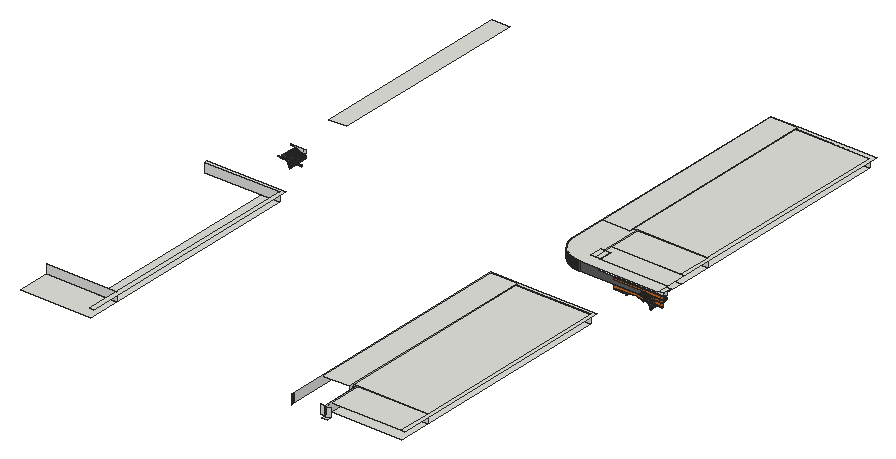
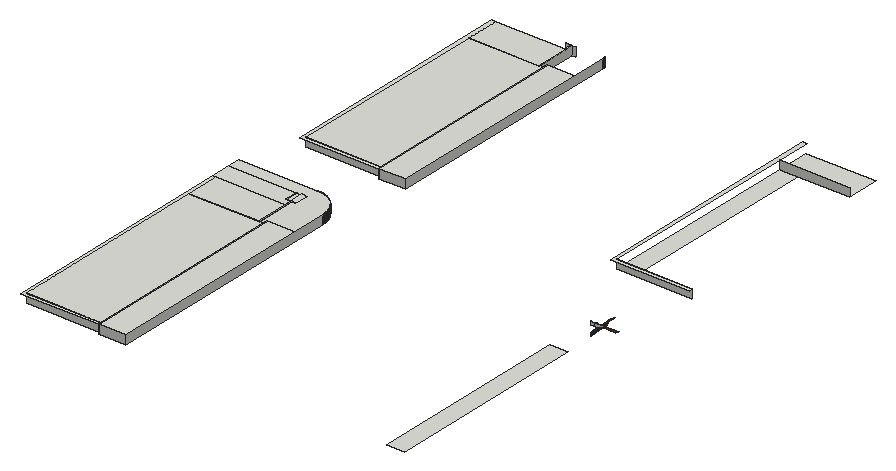
# SketchUp Ruby script. Lengths in inches.
U = 1.inch
M = Sketchup.active_model
def pt(a) = Geom::Point3d.new(a.map { |v| v * U })
def face(e, loops, mat)
  f = e.add_face(loops[0].map { |a| pt(a) })
  loops[1..].each { |l| e.add_face(l.map { |a| pt(a) }).erase! }
  f.material = f.back_material = mat if mat
  f
end
# faces: each face lists its corners as indices into pts; further lists are holes
def faces(e, pts, list, mat = nil) = list.each { |f| face(e, (f[0].is_a?(Array) ? f : [f]).map { |l| l.map { |i| pts[i] } }, mat) }
# xy, xz, yz: faces in a plane at the given z, y or x. An outline is a flat list of corners, or four numbers for a rectangle; further outlines are holes
def ring(l) = l.size == 4 ? [[l[0], l[1]], [l[2], l[1]], [l[2], l[3]], [l[0], l[3]]] : l.each_slice(2).to_a
def flat(e, list, mat, &to3) = list.each { |f| face(e, (f[0].is_a?(Array) ? f : [f]).map { |l| ring(l).map { |u, v| to3.(u, v) } }, mat) }
def xy(e, z, list, mat = nil) = flat(e, list, mat) { |x, y| [x, y, z] }
def xz(e, y, list, mat = nil) = flat(e, list, mat) { |x, z| [x, y, z] }
def yz(e, x, list, mat = nil) = flat(e, list, mat) { |y, z| [x, y, z] }
def lines(e, pts, list) = list.each { |a, b| e.add_line(pt(pts[a]), pt(pts[b])) }
# prism: a flat outline (further loops are holes) pulled along v
def prism(e, loops, v, mat = nil)
  f = face(e, loops, mat); d = Geom::Vector3d.new(v.map { |x| x * U })
  f.pushpull(f.normal.samedirection?(d) ? d.length : -d.length)
end
def box(e, o, s, mat = nil) = prism(e, [[o, [o[0] + s[0], o[1], o[2]], [o[0] + s[0], o[1] + s[1], o[2]], [o[0], o[1] + s[1], o[2]]]], [0, 0, s[2]], mat)
def at(x, y, z, deg = 0) = Geom::Transformation.translation(pt([x, y, z])) * Geom::Transformation.rotation(ORIGIN, Z_AXIS, deg.degrees)
def axes(o, x, y, z) = Geom::Transformation.new([*x, 0, *y, 0, *z, 0, *pt(o).to_a, 1])
def part(name) = M.definitions.add(name)
# library, detail: a bought-in or finely detailed component or shape, given as its bounding box
def library(name, o, s) = part(name).tap { |d| box(d.entities, o, s) }
def detail(e, o, s) = box(e.add_group.entities, o, s)
def put(e, d, t, mat = nil) = e.add_instance(d, t).tap { |i| i.material = mat if mat }
def group(e, t, mat = nil) = e.add_group.tap { |g| g.transformation = t; g.material = mat if mat }.entities
root = M.entities
M.materials.add("[0041_Chocolate]").color = [210, 105, 30]
M.materials.add("[Color M06]").color = [84, 84, 84]
xy(root,385.02,[[1533.33,971.36,1577.46,972.36],[2230.65,971.36,2260.14,972.36],[2287.96,971.36,2332.08,972.36]],"[0041_Chocolate]")
xy(root,386.9375,[[1528.37,971.36,1577.46,972.36],[2230.65,971.36,2265.11,972.36],[2282.99,971.36,2332.08,972.36]],"[0041_Chocolate]")
xy(root,391.89,[[2230.65,971.36,2332.08,972.36]],"[0041_Chocolate]")
xy(root,393.8125,[[2230.65,971.36,2332.08,972.36]],"[0041_Chocolate]")
xy(root,395.26,[[2230.65,993.35,2309.9,1001.16]])
xy(root,398.77,[[2230.65,971.36,2332.08,972.36]],"[0041_Chocolate]")
xy(root,400.6875,[[2230.65,971.36,2332.08,972.36]],"[0041_Chocolate]")
xy(root,402.64,[[2146.71,312.8125,2158.24,321.34],[1496.21,337.5625,1643.23,406.38],[2146.71,337.5625,2293.73,406.38],[2145.53,399.07,2146.71,406.38],[1606.23,406.38,1643.23,830.91],
  [2137,406.38,2145.53,830.91],[2145.53,406.38,2256.73,830.91],[2256.73,406.38,2293.73,830.91],[2230.65,991.23,2291.86,993.35],[2323.46,993.35,2326.17,993.35,2326.17,1028.46,2179.15,1028.46,2179.15,1012.23,2190.68,1012.23,2190.68,996.48,2230.65,996.48,2230.65,1003.71,2323.46,1003.71],
  [2230.65,993.35,2323.46,1003.71],[2169.44,996.48,2179.15,1003.71],[2179.15,996.48,2190.68,1003.71],[2169.44,1003.71,2179.15,1012.23],[2179.15,1003.71,2190.68,1012.23],
  [2179.15,1028.46,2326.17,1097.28],[2177.96,1089.96,2179.15,1097.28],[1534.54,1097.28,1571.54,1521.81],[2169.44,1097.28,2177.96,1521.81],[2177.96,1097.28,2289.17,1521.81],
  [2289.17,1097.28,2326.17,1521.81]])
xy(root,402.64,[[2168.39,958.64,2166.9,958.66,2165.41,958.72,2163.93,958.82,2162.44,958.96,2160.96,959.13,2159.49,959.34,2158.02,959.6,2156.5625,959.89,2155.11,960.22,2153.67,960.58,2152.23,960.99,2150.8125,961.43,2149.4,961.91,2148,962.42,2146.62,962.97,2145.25,963.5625,2143.9,964.1875,2142.5625,964.84,2141.25,965.54,2139.95,966.27,2138.67,967.03,2137.41,967.82,2136.17,968.65,2134.95,969.51,2133.76,970.4,2132.59,971.32,2131.44,972.27,2130.32,973.26,2129.23,974.27,2128.16,975.31,2127.125,976.37,2126.11,977.47,2125.13,978.59,2124.18,979.73,2123.26,980.9,2122.37,982.09,2121.51,983.31,2120.68,984.55,2119.89,985.81,2119.125,987.09,2118.4,988.39,2117.7,989.71,2117.04,991.04,2116.42,992.39,2115.83,993.76,2115.28,995.14,2114.77,996.54,2114.29,997.95,2113.85,999.375,2113.44,1000.81,2113.07,1002.25,2112.75,1003.7,2112.46,1005.16,2112.2,1006.63,2111.99,1008.11,2111.8125,1009.58,2111.68,1011.07,2111.58,1012.55,2111.52,1014.04,2111.5,1015.53,2111.5,1529.04,2169.44,1529.04,2169.44,996.48,2190.68,996.48,2190.68,978.84,2230.65,978.84,2230.65,991.23,2291.86,991.23,2291.86,958.64]],"[Color M06]")
xy(root,405.64,[[2230.65,971.36,2332.08,972.36]],"[0041_Chocolate]")
xy(root,411.82,[[2230.65,972.36,2332.08,993.35]])
xy(root,421.25,[[2145.53,321.34,2146.71,406.38],[2146.71,321.34,2148.59,321.34,2148.59,336.27,2293.73,336.27,2293.73,406.38,2146.71,406.38],[1643.23,336.27,1650.02,336.27,1650.02,838.14,1486.5,838.14,1486.5,830.91,1643.23,830.91],[2293.73,336.27,2300.52,336.27,2300.52,838.14,2137,838.14,2137,830.91,2293.73,830.91],[2079.07,397.86,2137,838.14],
  [2137,406.38,2293.73,830.91],[2168.39,958.64,2332.96,958.64,2332.96,983.34,2169.44,983.34,2169.44,1012.23,2177.96,1012.23,2177.96,1097.28,2169.44,1097.28,2169.44,1088.75,2111.5,1088.75,2111.5,1015.53,2111.52,1014.04,2111.58,1012.55,2111.68,1011.07,2111.8125,1009.58,2111.99,1008.11,2112.2,1006.63,2112.46,1005.16,2112.75,1003.7,2113.07,1002.25,2113.44,1000.81,2113.85,999.375,2114.29,997.95,2114.77,996.54,2115.28,995.14,2115.83,993.76,2116.42,992.39,2117.04,991.04,2117.7,989.71,2118.4,988.39,2119.125,987.09,2119.89,985.81,2120.68,984.55,2121.51,983.31,2122.37,982.09,2123.26,980.9,2124.18,979.73,2125.13,978.59,2126.11,977.47,2127.125,976.37,2128.16,975.31,2129.23,974.27,2130.32,973.26,2131.44,972.27,2132.59,971.32,2133.76,970.4,2134.95,969.51,2136.17,968.65,2137.41,967.82,2138.67,967.03,2139.95,966.27,2141.25,965.54,2142.5625,964.84,2143.9,964.1875,2145.25,963.5625,2146.62,962.97,2148,962.42,2149.4,961.91,2150.8125,961.43,2152.23,960.99,2153.67,960.58,2155.11,960.22,2156.5625,959.89,2158.02,959.6,2159.49,959.34,2160.96,959.13,2162.44,958.96,2163.93,958.82,2165.41,958.72,2166.9,958.66],[2169.44,983.34,2181.03,1012.23],[2181.03,983.34,2190.68,1012.23],[2190.68,983.34,2332.96,983.34,2332.96,1027.17,2181.03,1027.17,2181.03,1012.23,2190.68,1012.23],
  [2177.96,1012.23,2179.15,1097.28],[2179.15,1012.23,2181.03,1012.23,2181.03,1027.17,2326.17,1027.17,2326.17,1097.28,2179.15,1097.28],[2326.17,1027.17,2332.96,1027.17,2332.96,1529.04,2169.44,1529.04,2169.44,1521.81,2326.17,1521.81],[2111.5,1088.75,2169.44,1529.04],[2169.44,1097.28,2326.17,1521.81]])
xz(root,321.34,[[2137,402.64,2145.53,421.25],[2145.53,402.64,2146.71,421.25],[2146.71,402.64,2148.59,421.25],[2148.59,402.64,2158.24,421.25]])
xz(root,406.38,[[1496.21,402.64,1643.23,421.25],[2137,402.64,2145.53,421.25],[2145.53,402.64,2146.71,421.25],[2146.71,402.64,2293.73,421.25]])
xz(root,830.91,[[1486.5,402.64,1643.23,421.25],[2137,402.64,2293.73,421.25]])
xz(root,838.14,[[2079.07,402.64,2137,421.25]])
xz(root,971.36,[[2230.65,386.9375,2265.11,386.9375,2269.94,388.23,2278.13,388.24,2282.99,386.9375,2332.08,386.9375,2332.08,391.89,2230.65,391.89],[2230.65,393.8125,2332.08,398.77],[2230.65,400.6875,2332.08,405.64]],"[0041_Chocolate]")
xz(root,972.36,[[2230.65,405.64,2332.08,407.5625],[2230.65,407.5625,2332.08,411.82],[2230.65,411.82,2332.08,412.52]])
xz(root,972.36,[[1533.33,385.02,1577.46,385.02,1577.46,386.9375,1528.37,386.9375,1531.41,386.125],[2230.65,385.02,2260.14,385.02,2262.03,386.11,2265.11,386.9375,2230.65,386.9375],[2287.96,385.02,2332.08,385.02,2332.08,386.9375,2282.99,386.9375,2286.04,386.125],[2230.65,391.89,2332.08,393.8125],[2230.65,398.77,2332.08,400.6875]],"[0041_Chocolate]")
xz(root,993.35,[[1555.27,395.26,1562.99,395.26,1562.99,402.64,1537.23,402.64,1537.91,402.625,1538.58,402.6,1539.25,402.56,1539.92,402.49,1540.59,402.41,1541.26,402.32,1541.93,402.2,1542.59,402.07,1543.25,401.92,1543.9,401.76,1544.55,401.57,1545.19,401.375,1545.83,401.16,1546.46,400.92,1547.09,400.67,1547.71,400.41,1548.32,400.125,1548.93,399.83,1549.52,399.51,1550.11,399.18,1550.69,398.84,1551.26,398.48,1551.82,398.1,1552.37,397.72,1552.91,397.3125,1553.44,396.89,1553.96,396.46,1554.47,396.02,1554.96,395.5625],[1562.99,395.26,1568.84,402.64],[2230.65,395.26,2309.9,395.26,2309.59,395.5625,2309.09,396.02,2308.59,396.46,2308.07,396.89,2307.54,397.3125,2307,397.72,2306.45,398.1,2305.89,398.48,2305.32,398.84,2304.74,399.18,2304.15,399.51,2303.55,399.83,2302.95,400.125,2302.33,400.41,2301.71,400.67,2301.09,400.92,2300.46,401.16,2299.82,401.375,2299.17,401.57,2298.52,401.76,2297.87,401.92,2297.21,402.07,2296.55,402.2,2295.89,402.32,2295.22,402.41,2294.55,402.49,2293.88,402.56,2293.2,402.6,2292.53,402.625,2291.86,402.64,2230.65,402.64],[2309.9,395.26,2317.62,395.26,2317.62,402.64,2291.86,402.64,2292.53,402.625,2293.2,402.6,2293.88,402.56,2294.55,402.49,2295.22,402.41,2295.89,402.32,2296.55,402.2,2297.21,402.07,2297.87,401.92,2298.52,401.76,2299.17,401.57,2299.82,401.375,2300.46,401.16,2301.09,400.92,2301.71,400.67,2302.33,400.41,2302.95,400.125,2303.55,399.83,2304.15,399.51,2304.74,399.18,2305.32,398.84,2305.89,398.48,2306.45,398.1,2307,397.72,2307.54,397.3125,2308.07,396.89,2308.59,396.46,2309.09,396.02,2309.59,395.5625],[2317.62,395.26,2323.46,402.64],
  [2230.65,402.64,2317.62,411.82]])
xz(root,1012.23,[[2169.44,402.64,2177.96,421.25],[2177.96,402.64,2179.15,421.25],[2179.15,402.64,2181.03,421.25],[2181.03,402.64,2190.68,421.25]])
xz(root,1097.28,[[2169.44,402.64,2177.96,421.25],[2177.96,402.64,2179.15,421.25],[2179.15,402.64,2326.17,421.25]])
xz(root,1521.81,[[2169.44,402.64,2326.17,421.25]])
xz(root,1529.04,[[2111.5,402.64,2169.44,421.25]])
yz(root,2079.07,[[324.64,402.64,838.14,421.25]])
yz(root,2111.5,[[1015.53,402.64,1529.04,421.25]])
yz(root,2137,[[397.86,402.64,406.38,421.25],[406.38,402.64,830.91,421.25],[830.91,402.64,838.14,421.25]])
yz(root,2146.71,[[321.34,402.64,406.38,421.25]])
yz(root,2169.44,[[1088.75,402.64,1097.28,421.25],[1097.28,402.64,1521.81,421.25],[1521.81,402.64,1529.04,421.25]])
yz(root,2179.15,[[1012.23,402.64,1097.28,421.25]])
yz(root,2190.68,[[983.34,402.64,1012.23,421.25]])
yz(root,2230.65,[[991.23,395.26,993.35,402.64],[993.35,395.26,996.48,402.64]])
p = [[1562.56,958.64,381.57],[1562.56,993.35,381.57],[1562.67,993.35,380.9],[1562.67,958.64,380.9],[2317.19,958.64,381.57],[2317.19,993.35,381.57],
  [2317.3,993.35,380.9],[2317.3,958.64,380.9],[1562.67,1001.16,380.9],[1562.56,1001.16,381.57],[2317.3,1001.16,380.9],[2317.19,1001.16,381.57],
  [1562.43,958.64,382.23],[1562.43,993.35,382.23],[2317.05,958.64,382.23],[2317.05,993.35,382.23],[1562.43,1001.16,382.23],[2317.05,1001.16,382.23],
  [2260.14,986.55,385.02],[2260.14,972.36,385.02],[2260.14,971.36,385.02],[2254.94,971.36,382.01],[2254.94,986.55,382.01],[2293.13,986.55,382.03],
  [2293.13,971.36,382.03],[2287.96,971.36,385.02],[2287.96,972.36,385.02],[2287.96,986.55,385.02],[1562.28,958.64,382.89],[1562.28,993.35,382.89],
  [2316.9,958.64,382.89],[2316.9,993.35,382.89],[1562.28,1001.16,382.89],[2316.9,1001.16,382.89],[1562.11,958.64,383.54],[1562.11,993.35,383.54],
  [2316.74,958.64,383.54],[2316.74,993.35,383.54],[1562.11,1001.16,383.54],[2316.74,1001.16,383.54],[1561.93,958.64,384.19],[1561.93,993.35,384.19],
  [1562.09,993.35,383.64],[2316.56,958.64,384.19],[2316.56,993.35,384.19],[2316.71,993.35,383.64],[1562.09,1001.16,383.64],[2316.71,1001.16,383.64],
  [1561.93,1001.16,384.19],[2316.56,1001.16,384.19],[1561.73,958.64,384.84],[1561.73,993.35,384.84],[2316.36,958.64,384.84],[2316.36,993.35,384.84],
  [1561.73,1001.16,384.84],[2316.36,1001.16,384.84],[1561.51,958.64,385.47],[1561.51,993.35,385.47],[2316.14,958.64,385.47],[2316.14,993.35,385.47],
  [1561.51,1001.16,385.47],[2316.14,1001.16,385.47],[2262.03,972.36,386.11],[2262.03,986.55,386.11],[2286.04,972.36,386.125],[2286.04,986.55,386.125],
  [1561.28,958.64,386.11],[1561.28,993.35,386.11],[1561.41,993.35,385.76],[2315.91,958.64,386.11],[2315.91,993.35,386.11],[2316.03,993.35,385.76],
  [1561.41,1001.16,385.76],[2316.03,1001.16,385.76],[1561.28,1001.16,386.11],[2315.91,1001.16,386.11],[1561.03,958.64,386.73],[1561.03,993.35,386.73],
  [2315.66,958.64,386.73],[2315.66,993.35,386.73],[2265.11,972.36,386.9375],[2265.11,986.55,386.9375],[2282.99,972.36,386.9375],[2282.99,986.55,386.9375],
  [1561.03,1001.16,386.73],[2315.66,1001.16,386.73],[1560.76,958.64,387.35],[1560.76,993.35,387.35],[2315.39,958.64,387.35],[2315.39,993.35,387.35],
  [1560.76,1001.16,387.35],[2315.39,1001.16,387.35],[2269.94,986.55,388.23],[2269.94,971.36,388.23],[2265.11,971.36,386.9375],[2282.99,971.36,386.9375],
  [2278.13,971.36,388.24],[2278.13,986.55,388.24],[1560.48,958.64,387.96],[1560.48,993.35,387.96],[2315.11,958.64,387.96],[2315.11,993.35,387.96],
  [1560.48,1001.16,387.96],[2315.11,1001.16,387.96],[1560.18,958.64,388.57],[1560.18,993.35,388.57],[2314.81,958.64,388.57],[2314.81,993.35,388.57],
  [1560.18,1001.16,388.57],[2314.81,1001.16,388.57],[1559.87,958.64,389.17],[1559.87,993.35,389.17],[2314.49,958.64,389.17],[2314.49,993.35,389.17],
  [1559.87,1001.16,389.17],[2314.49,1001.16,389.17],[1559.54,958.64,389.76],[1559.54,993.35,389.76],[2314.17,958.64,389.76],[2314.17,993.35,389.76],
  [1559.54,1001.16,389.76],[2314.17,1001.16,389.76],[1559.2,958.64,390.33],[1559.2,993.35,390.33],[2313.82,958.64,390.33],[2313.82,993.35,390.33],
  [1559.2,1001.16,390.33],[2313.82,1001.16,390.33],[1558.84,958.64,390.9],[1558.84,993.35,390.9],[2313.46,958.64,390.9],[2313.46,993.35,390.9],
  [1558.84,1001.16,390.9],[2313.46,1001.16,390.9],[1558.46,958.64,391.47],[1558.46,993.35,391.47],[2313.09,958.64,391.47],[2313.09,993.35,391.47],
  [1558.46,1001.16,391.47],[2313.09,1001.16,391.47],[1558.07,958.64,392.02],[1558.07,993.35,392.02],[2312.7,958.64,392.02],[2312.7,993.35,392.02],
  [1558.07,1001.16,392.02],[2312.7,1001.16,392.02],[1557.67,958.64,392.56],[1557.67,993.35,392.56],[2312.29,958.64,392.56],[2312.29,993.35,392.56],
  [1557.67,1001.16,392.56],[2312.29,1001.16,392.56],[1557.25,958.64,393.09],[1557.25,993.35,393.09],[2311.875,958.64,393.09],[2311.875,993.35,393.09],
  [1557.25,1001.16,393.09],[2311.875,1001.16,393.09],[1556.82,958.64,393.6],[1556.82,993.35,393.6],[1557.21,993.35,393.14],[2311.44,958.64,393.6],
  [2311.44,993.35,393.6],[2311.84,993.35,393.14],[1557.21,1001.16,393.14],[1556.82,1001.16,393.6],[2311.84,1001.16,393.14],[2311.44,1001.16,393.6],
  [1556.375,958.64,394.11],[1556.375,993.35,394.11],[2311,958.64,394.11],[2311,993.35,394.11],[1556.375,1001.16,394.11],[2311,1001.16,394.11],
  [1555.92,958.64,394.61],[1555.92,993.35,394.61],[2310.54,958.64,394.61],[2310.54,993.35,394.61],[1555.92,1001.16,394.61],[2310.54,1001.16,394.61],
  [1555.45,958.64,395.09],[1555.45,993.35,395.09],[2310.07,958.64,395.09],[2310.07,993.35,395.09],[1555.45,1001.16,395.09],[2310.07,1001.16,395.09],
  [1554.96,958.64,395.5625],[1554.96,991.23,395.5625],[1555.27,991.23,395.26],[1555.27,993.35,395.26],[2309.59,958.64,395.5625],[2309.59,991.23,395.5625],
  [2309.9,991.23,395.26],[2309.9,993.35,395.26],[1555.27,1001.16,395.26],[2309.9,1001.16,395.26],[1554.96,993.35,395.5625],[2309.59,993.35,395.5625],
  [1554.47,958.64,396.02],[1554.47,991.23,396.02],[2309.09,958.64,396.02],[2309.09,991.23,396.02],[1554.47,993.35,396.02],[2309.09,993.35,396.02],
  [1553.96,958.64,396.46],[1553.96,991.23,396.46],[2308.59,958.64,396.46],[2308.59,991.23,396.46],[1553.96,993.35,396.46],[2308.59,993.35,396.46],
  [1553.44,958.64,396.89],[1553.44,991.23,396.89],[2308.07,958.64,396.89],[2308.07,991.23,396.89],[1553.44,993.35,396.89],[2308.07,993.35,396.89],
  [1552.91,958.64,397.3125],[1552.91,991.23,397.3125],[2307.54,958.64,397.3125],[2307.54,991.23,397.3125],[1552.91,993.35,397.3125],[2307.54,993.35,397.3125],
  [1552.37,958.64,397.72],[1552.37,991.23,397.72],[2307,958.64,397.72],[2307,991.23,397.72],[1552.37,993.35,397.72],[2307,993.35,397.72],
  [1551.82,958.64,398.1],[1551.82,991.23,398.1],[2306.45,958.64,398.1],[2306.45,991.23,398.1],[1551.82,993.35,398.1],[2306.45,993.35,398.1],
  [1551.26,958.64,398.48],[1551.26,991.23,398.48],[2305.89,958.64,398.48],[2305.89,991.23,398.48],[1551.26,993.35,398.48],[2305.89,993.35,398.48],
  [1550.69,958.64,398.84],[1550.69,991.23,398.84],[2305.32,958.64,398.84],[2305.32,991.23,398.84],[1550.69,993.35,398.84],[2305.32,993.35,398.84],
  [1550.11,958.64,399.18],[1550.11,991.23,399.18],[2304.74,958.64,399.18],[2304.74,991.23,399.18],[1550.11,993.35,399.18],[2304.74,993.35,399.18],
  [1549.52,958.64,399.51],[1549.52,991.23,399.51],[2304.15,958.64,399.51],[2304.15,991.23,399.51],[1549.52,993.35,399.51],[2304.15,993.35,399.51],
  [1548.93,958.64,399.83],[1548.93,991.23,399.83],[2303.55,958.64,399.83],[2303.55,991.23,399.83],[1548.93,993.35,399.83],[2303.55,993.35,399.83],
  [1548.32,958.64,400.125],[1548.32,991.23,400.125],[2302.95,958.64,400.125],[2302.95,991.23,400.125],[1548.32,993.35,400.125],[2302.95,993.35,400.125],
  [1547.71,958.64,400.41],[1547.71,991.23,400.41],[2302.33,958.64,400.41],[2302.33,991.23,400.41],[1547.71,993.35,400.41],[2302.33,993.35,400.41],
  [1547.09,958.64,400.67],[1547.09,991.23,400.67],[2301.71,958.64,400.67],[2301.71,991.23,400.67],[1547.09,993.35,400.67],[2301.71,993.35,400.67],
  [2301.09,958.64,400.92],[2301.09,991.23,400.92],[2301.09,993.35,400.92],[2300.46,958.64,401.16],[2300.46,991.23,401.16],[2300.46,993.35,401.16],
  [2299.82,958.64,401.375],[2299.82,991.23,401.375],[2299.82,993.35,401.375],[2299.17,958.64,401.57],[2299.17,991.23,401.57],[2299.17,993.35,401.57],
  [2298.52,958.64,401.76],[2298.52,991.23,401.76],[2298.52,993.35,401.76],[2297.87,958.64,401.92],[2297.87,991.23,401.92],[2297.87,993.35,401.92],
  [2297.21,958.64,402.07],[2297.21,991.23,402.07],[2297.21,993.35,402.07],[2296.55,958.64,402.2],[2296.55,991.23,402.2],[2296.55,993.35,402.2],
  [2295.89,958.64,402.32],[2295.89,991.23,402.32],[2295.89,993.35,402.32],[2295.22,958.64,402.41],[2295.22,991.23,402.41],[2295.22,993.35,402.41],
  [2294.55,958.64,402.49],[2294.55,991.23,402.49],[2294.55,993.35,402.49],[2293.88,958.64,402.56],[2293.88,991.23,402.56],[2293.88,993.35,402.56],
  [2079.55,317.21,421.25],[2079.375,318.69,421.25],[2079.375,318.69,402.64],[2079.55,317.21,402.64],[2079.24,320.17,421.25],[2079.24,320.17,402.64],
  [2079.14,321.66,421.25],[2079.14,321.66,402.64],[2079.08,323.15,421.25],[2079.08,323.15,402.64],[2079.07,324.64,421.25],[2079.07,324.64,402.64],
  [2168.39,958.64,421.25],[2166.9,958.66,421.25],[2166.9,958.66,402.64],[2168.39,958.64,402.64],[2291.86,958.64,402.64],[2291.86,991.23,402.64],
  [2292.53,991.23,402.625],[2292.53,958.64,402.625],[2293.2,991.23,402.6],[2293.2,958.64,402.6],[2165.41,958.72,421.25],[2163.93,958.82,421.25],
  [2163.93,958.82,402.64],[2165.41,958.72,402.64],[2162.44,958.96,421.25],[2162.44,958.96,402.64],[2160.96,959.13,421.25],[2160.96,959.13,402.64],
  [2159.49,959.34,421.25],[2159.49,959.34,402.64],[2158.02,959.6,421.25],[2158.02,959.6,402.64],[2156.5625,959.89,421.25],[2156.5625,959.89,402.64],
  [2155.11,960.22,421.25],[2155.11,960.22,402.64],[2153.67,960.58,421.25],[2153.67,960.58,402.64],[2152.23,960.99,421.25],[2152.23,960.99,402.64],
  [2150.8125,961.43,421.25],[2150.8125,961.43,402.64],[2149.4,961.91,421.25],[2149.4,961.91,402.64],[2148,962.42,421.25],[2148,962.42,402.64],
  [2146.62,962.97,421.25],[2146.62,962.97,402.64],[2145.25,963.5625,421.25],[2145.25,963.5625,402.64],[2143.9,964.1875,421.25],[2143.9,964.1875,402.64],
  [2142.5625,964.84,421.25],[2142.5625,964.84,402.64],[2141.25,965.54,421.25],[2141.25,965.54,402.64],[2139.95,966.27,421.25],[2139.95,966.27,402.64],
  [2138.67,967.03,421.25],[2138.67,967.03,402.64],[2137.41,967.82,421.25],[2137.41,967.82,402.64],[2136.17,968.65,421.25],[2136.17,968.65,402.64],
  [2134.95,969.51,421.25],[2134.95,969.51,402.64],[2133.76,970.4,421.25],[2133.76,970.4,402.64],[2132.59,971.32,421.25],[2132.59,971.32,402.64],
  [2131.44,972.27,421.25],[2131.44,972.27,402.64],[2130.32,973.26,421.25],[2130.32,973.26,402.64],[2129.23,974.27,421.25],[2129.23,974.27,402.64],
  [2128.16,975.31,421.25],[2128.16,975.31,402.64],[2127.125,976.37,421.25],[2127.125,976.37,402.64],[2126.11,977.47,421.25],[2126.11,977.47,402.64],
  [2125.13,978.59,421.25],[2125.13,978.59,402.64],[2124.18,979.73,421.25],[2124.18,979.73,402.64],[2123.26,980.9,421.25],[2123.26,980.9,402.64],
  [2122.37,982.09,421.25],[2122.37,982.09,402.64],[2121.51,983.31,421.25],[2121.51,983.31,402.64],[2120.68,984.55,421.25],[2120.68,984.55,402.64],
  [2119.89,985.81,421.25],[2119.89,985.81,402.64],[2119.125,987.09,421.25],[2119.125,987.09,402.64],[2118.4,988.39,421.25],[2118.4,988.39,402.64],
  [2117.7,989.71,421.25],[2117.7,989.71,402.64],[2117.04,991.04,421.25],[2117.04,991.04,402.64],[2116.42,992.39,421.25],[2116.42,992.39,402.64],
  [2291.86,993.35,402.64],[2292.53,993.35,402.625],[2293.2,993.35,402.6],[2115.83,993.76,421.25],[2115.83,993.76,402.64],[2115.28,995.14,421.25],
  [2115.28,995.14,402.64],[2114.77,996.54,421.25],[2114.77,996.54,402.64],[2114.29,997.95,421.25],[2114.29,997.95,402.64],[2113.85,999.375,421.25],
  [2113.85,999.375,402.64],[2113.44,1000.81,421.25],[2113.44,1000.81,402.64],[2113.07,1002.25,421.25],[2113.07,1002.25,402.64],[2112.75,1003.7,421.25],
  [2112.75,1003.7,402.64],[2112.46,1005.16,421.25],[2112.46,1005.16,402.64],[2112.2,1006.63,421.25],[2112.2,1006.63,402.64],[2111.99,1008.11,421.25],
  [2111.99,1008.11,402.64],[2111.8125,1009.58,421.25],[2111.8125,1009.58,402.64],[2111.68,1011.07,421.25],[2111.68,1011.07,402.64],[2111.58,1012.55,421.25],
  [2111.58,1012.55,402.64],[2111.52,1014.04,421.25],[2111.52,1014.04,402.64],[2111.5,1015.53,421.25],[2111.5,1015.53,402.64]]
faces(root,p,[[0,1,2,3],[4,5,6,7],[12,13,1,0],[14,15,5,4],[28,29,13,12],[30,31,15,14],[34,35,29,28],[36,37,31,30],
  [40,41,42,35,34],[43,44,45,37,36],[50,51,41,40],[52,53,44,43],[56,57,51,50],[58,59,53,52],[66,67,68,57,56],[69,70,71,59,58],
  [76,77,67,66],[78,79,70,69],[86,87,77,76],[88,89,79,78],[98,99,87,86],[100,101,89,88],[104,105,99,98],[106,107,101,100],
  [110,111,105,104],[112,113,107,106],[116,117,111,110],[118,119,113,112],[122,123,117,116],[124,125,119,118],[128,129,123,122],[130,131,125,124],
  [134,135,129,128],[136,137,131,130],[140,141,135,134],[142,143,137,136],[146,147,141,140],[148,149,143,142],[152,153,147,146],[154,155,149,148],
  [158,159,160,153,152],[161,162,163,155,154],[168,169,159,158],[170,171,162,161],[174,175,169,168],[176,177,171,170],[180,181,175,174],[182,183,177,176],
  [186,187,188,189,181,180],[190,191,192,193,183,182],[198,199,187,186],[200,201,191,190],[204,205,199,198],[206,207,201,200],[210,211,205,204],[212,213,207,206],
  [216,217,211,210],[218,219,213,212],[222,223,217,216],[224,225,219,218],[228,229,223,222],[230,231,225,224],[234,235,229,228],[236,237,231,230],
  [240,241,235,234],[242,243,237,236],[246,247,241,240],[248,249,243,242],[252,253,247,246],[254,255,249,248],[258,259,253,252],[260,261,255,254],
  [264,265,259,258],[266,267,261,260],[270,271,265,264],[272,273,267,266],[276,277,271,270],[278,279,273,272],[282,283,279,278],[285,286,283,282],
  [288,289,286,285],[291,292,289,288],[294,295,292,291],[297,298,295,294],[300,301,298,297],[303,304,301,300],[306,307,304,303],[309,310,307,306],
  [312,313,310,309],[315,316,313,312],[318,319,320,321],[319,322,323,320],[322,324,325,323],[324,326,327,325],[326,328,329,327],[330,331,332,333],
  [334,335,336,337],[337,336,338,339],[339,338,316,315],[340,341,342,343],[331,340,343,332],[341,344,345,342],[344,346,347,345],[346,348,349,347],
  [348,350,351,349],[350,352,353,351],[352,354,355,353],[354,356,357,355],[356,358,359,357],[358,360,361,359],[360,362,363,361],[362,364,365,363],
  [364,366,367,365],[366,368,369,367],[368,370,371,369],[370,372,373,371],[372,374,375,373],[374,376,377,375],[376,378,379,377],[378,380,381,379],
  [380,382,383,381],[382,384,385,383],[384,386,387,385],[386,388,389,387],[388,390,391,389],[390,392,393,391],[392,394,395,393],[394,396,397,395],
  [396,398,399,397],[398,400,401,399],[400,402,403,401],[402,404,405,403],[404,406,407,405],[406,408,409,407],[408,410,411,409],[410,412,413,411],
  [412,414,415,413],[414,416,417,415],[416,418,419,417],[418,420,421,419],[420,422,423,421],[422,424,425,423],[424,429,430,425],[429,431,432,430],
  [431,433,434,432],[433,435,436,434],[435,437,438,436],[437,439,440,438],[439,441,442,440],[441,443,444,442],[443,445,446,444],[445,447,448,446],
  [447,449,450,448],[449,451,452,450],[451,453,454,452],[453,455,456,454],[455,457,458,456],[457,459,460,458]],"[Color M06]")
faces(root,p,[[1,2,8,9],[5,6,10,11],[13,1,9,16],[15,5,11,17],[18,19,20,21,22],[23,24,25,26,27],[29,13,16,32],[31,15,17,33],
  [35,29,32,38],[37,31,33,39],[42,35,38,46],[45,37,39,47],[41,42,46,48],[44,45,47,49],[51,41,48,54],[53,44,49,55],
  [57,51,54,60],[59,53,55,61],[62,19,18,63],[26,64,65,27],[68,57,60,72],[71,59,61,73],[67,68,72,74],[70,71,73,75],
  [80,62,63,81],[64,82,83,65],[77,67,74,84],[79,70,75,85],[87,77,84,90],[89,79,85,91],[92,93,94,80,81],[83,82,95,96,97],
  [99,87,90,102],[101,89,91,103],[105,99,102,108],[107,101,103,109],[97,96,93,92],[111,105,108,114],[113,107,109,115],[117,111,114,120],
  [119,113,115,121],[123,117,120,126],[125,119,121,127],[129,123,126,132],[131,125,127,133],[135,129,132,138],[137,131,133,139],[141,135,138,144],
  [143,137,139,145],[147,141,144,150],[149,143,145,151],[153,147,150,156],[155,149,151,157],[159,160,164,165],[160,153,156,164],[162,163,166,167],
  [163,155,157,166],[169,159,165,172],[171,162,167,173],[175,169,172,178],[177,171,173,179],[181,175,178,184],[183,177,179,185],[189,181,184,194],
  [193,183,185,195],[196,189,188,187],[197,193,192,191],[202,196,187,199],[203,197,191,201],[208,202,199,205],[209,203,201,207],[214,208,205,211],
  [215,209,207,213],[220,214,211,217],[221,215,213,219],[226,220,217,223],[227,221,219,225],[232,226,223,229],[233,227,225,231],[238,232,229,235],
  [239,233,231,237],[244,238,235,241],[245,239,237,243],[250,244,241,247],[251,245,243,249],[256,250,247,253],[257,251,249,255],[262,256,253,259],
  [263,257,255,261],[268,262,259,265],[269,263,261,267],[274,268,265,271],[275,269,267,273],[280,274,271,277],[281,275,273,279],[284,281,279,283],
  [287,284,283,286],[290,287,286,289],[293,290,289,292],[296,293,292,295],[299,296,295,298],[302,299,298,301],[305,302,301,304],[308,305,304,307],
  [311,308,307,310],[314,311,310,313],[317,314,313,316],[426,427,336,335],[427,428,338,336],[428,317,316,338]])
